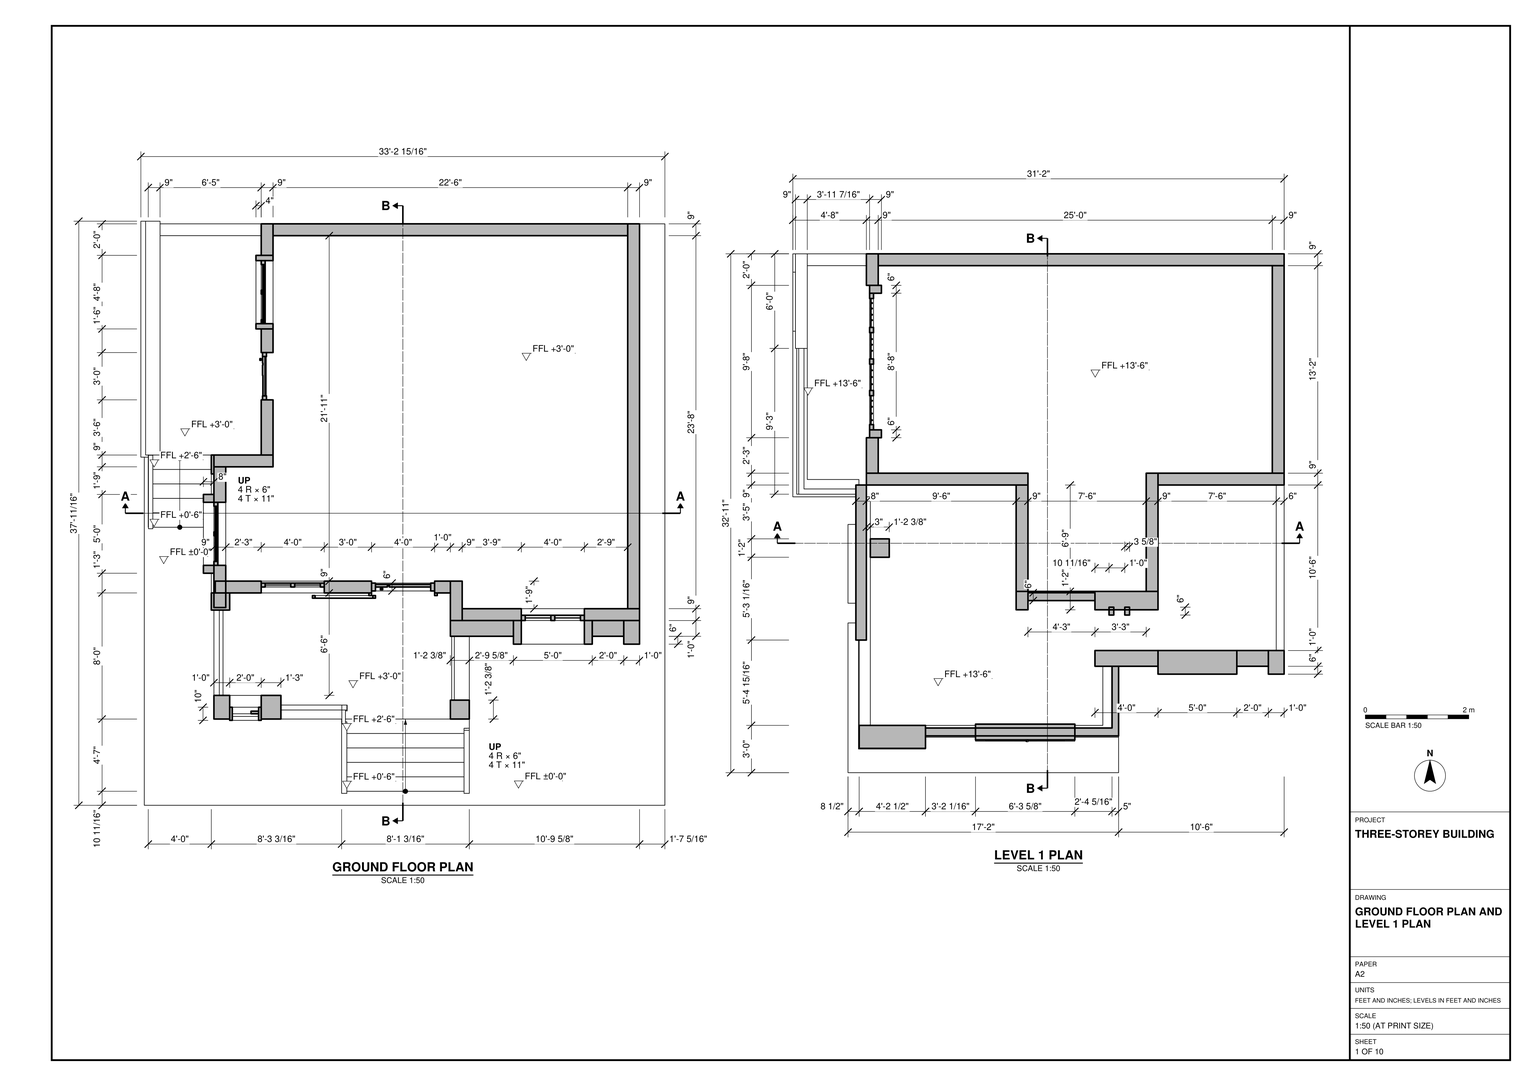
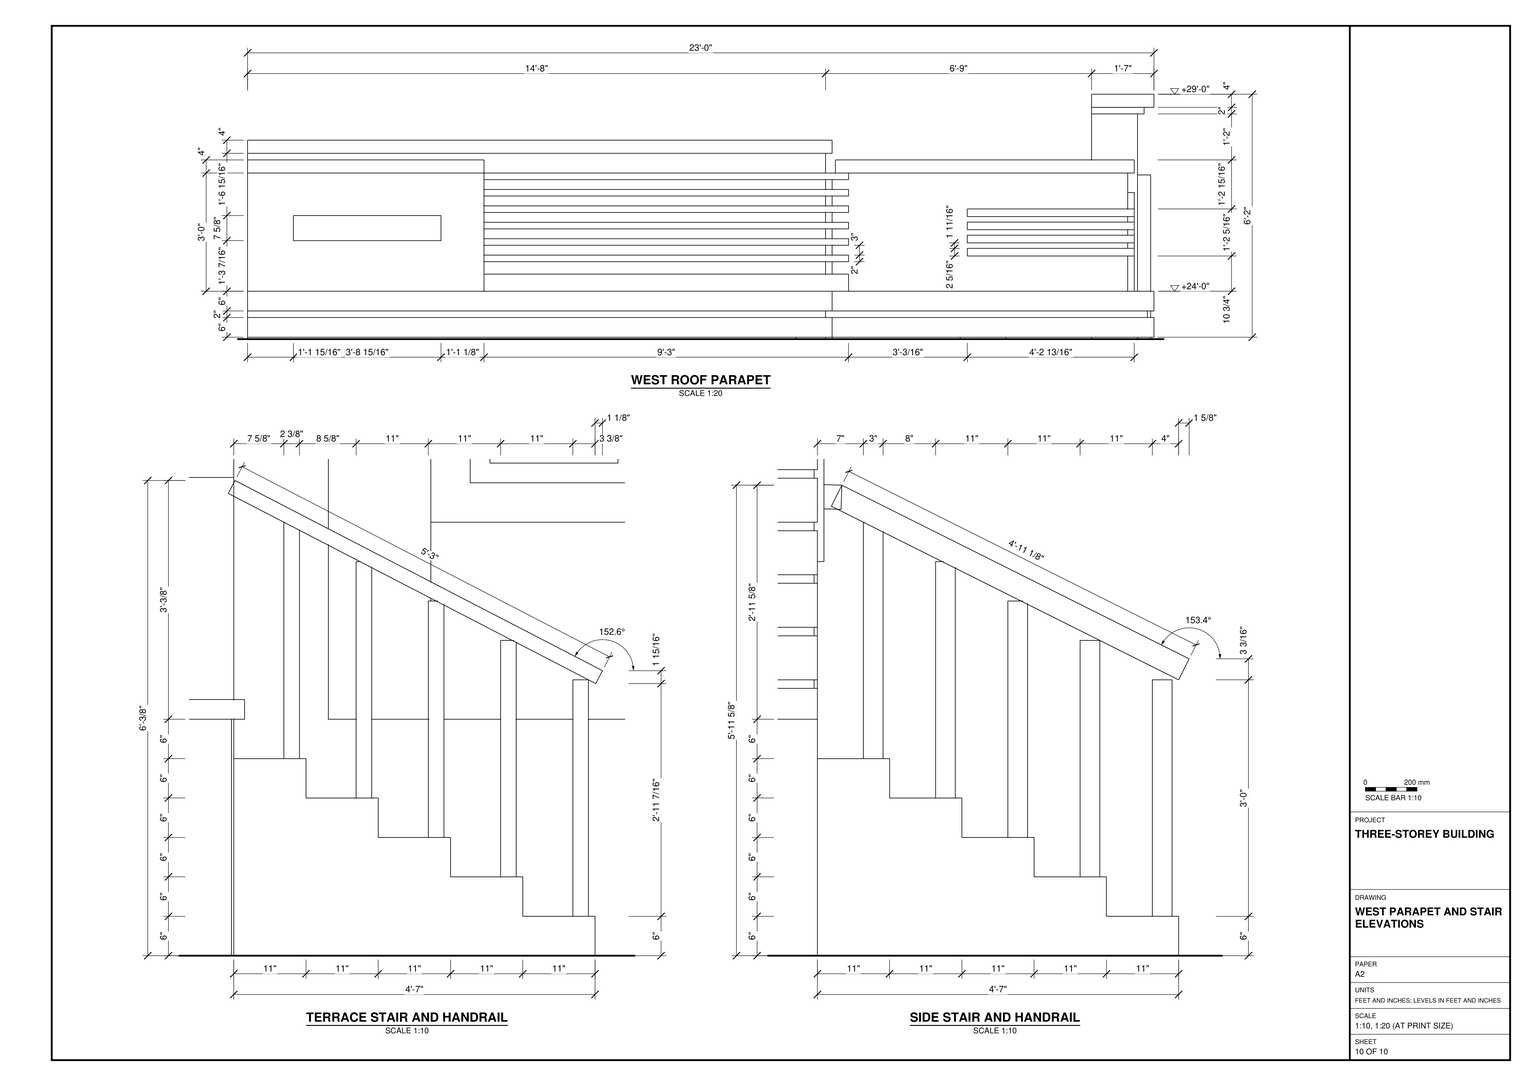
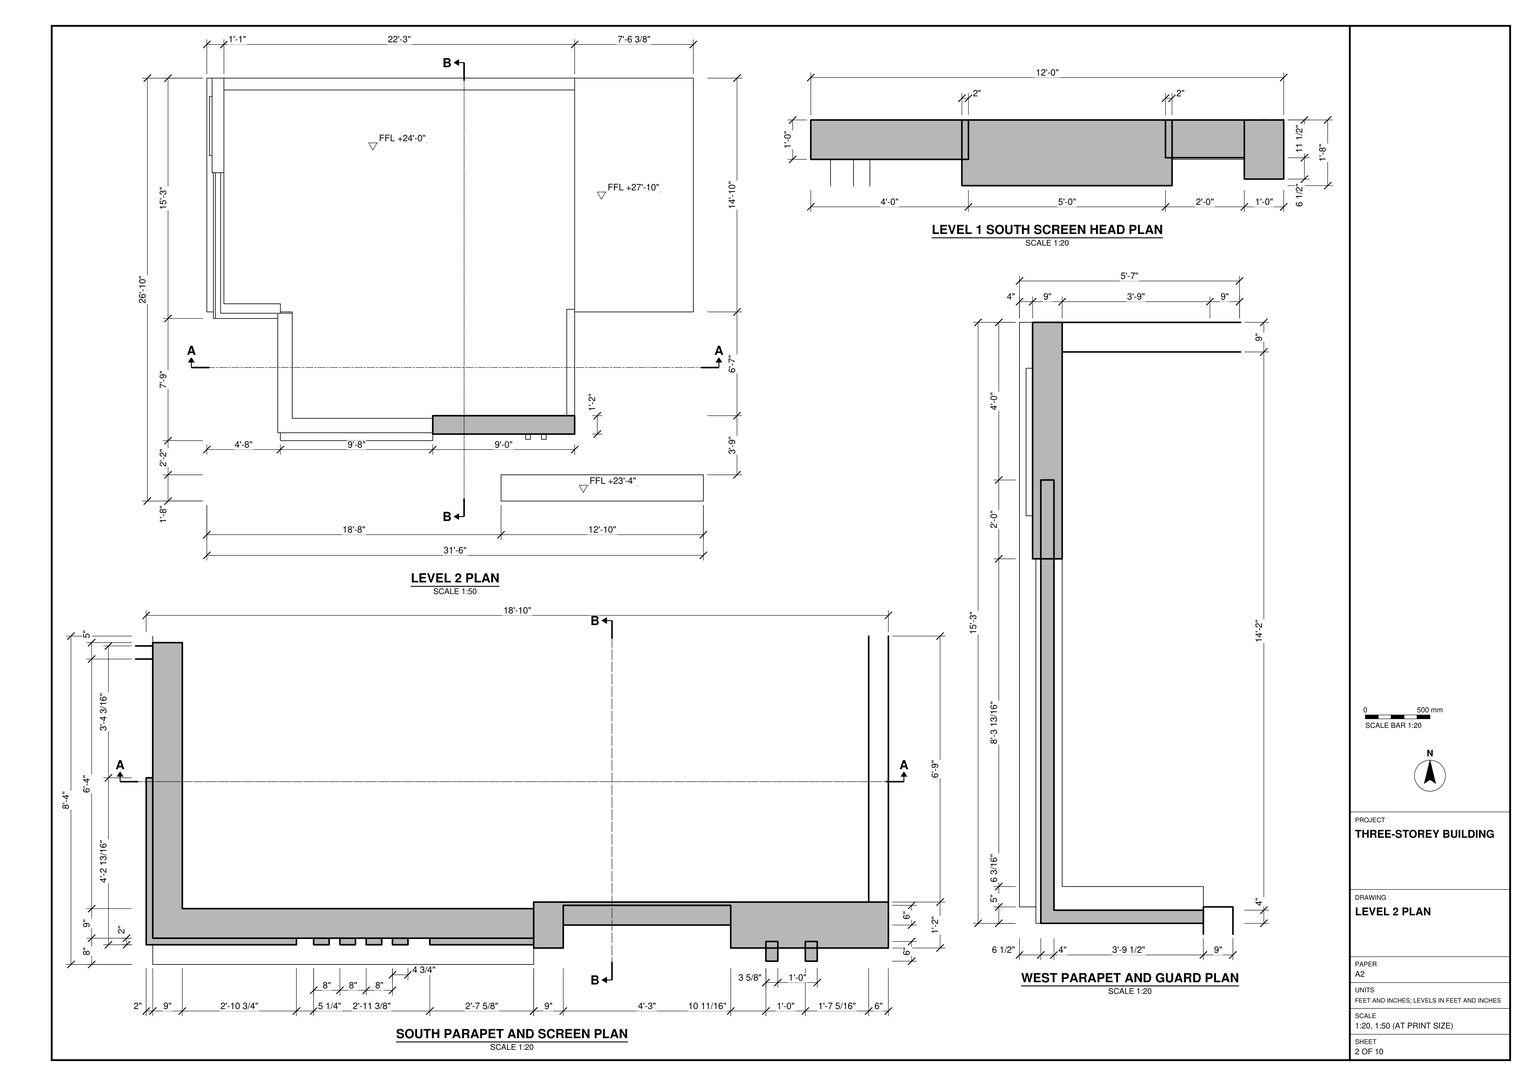
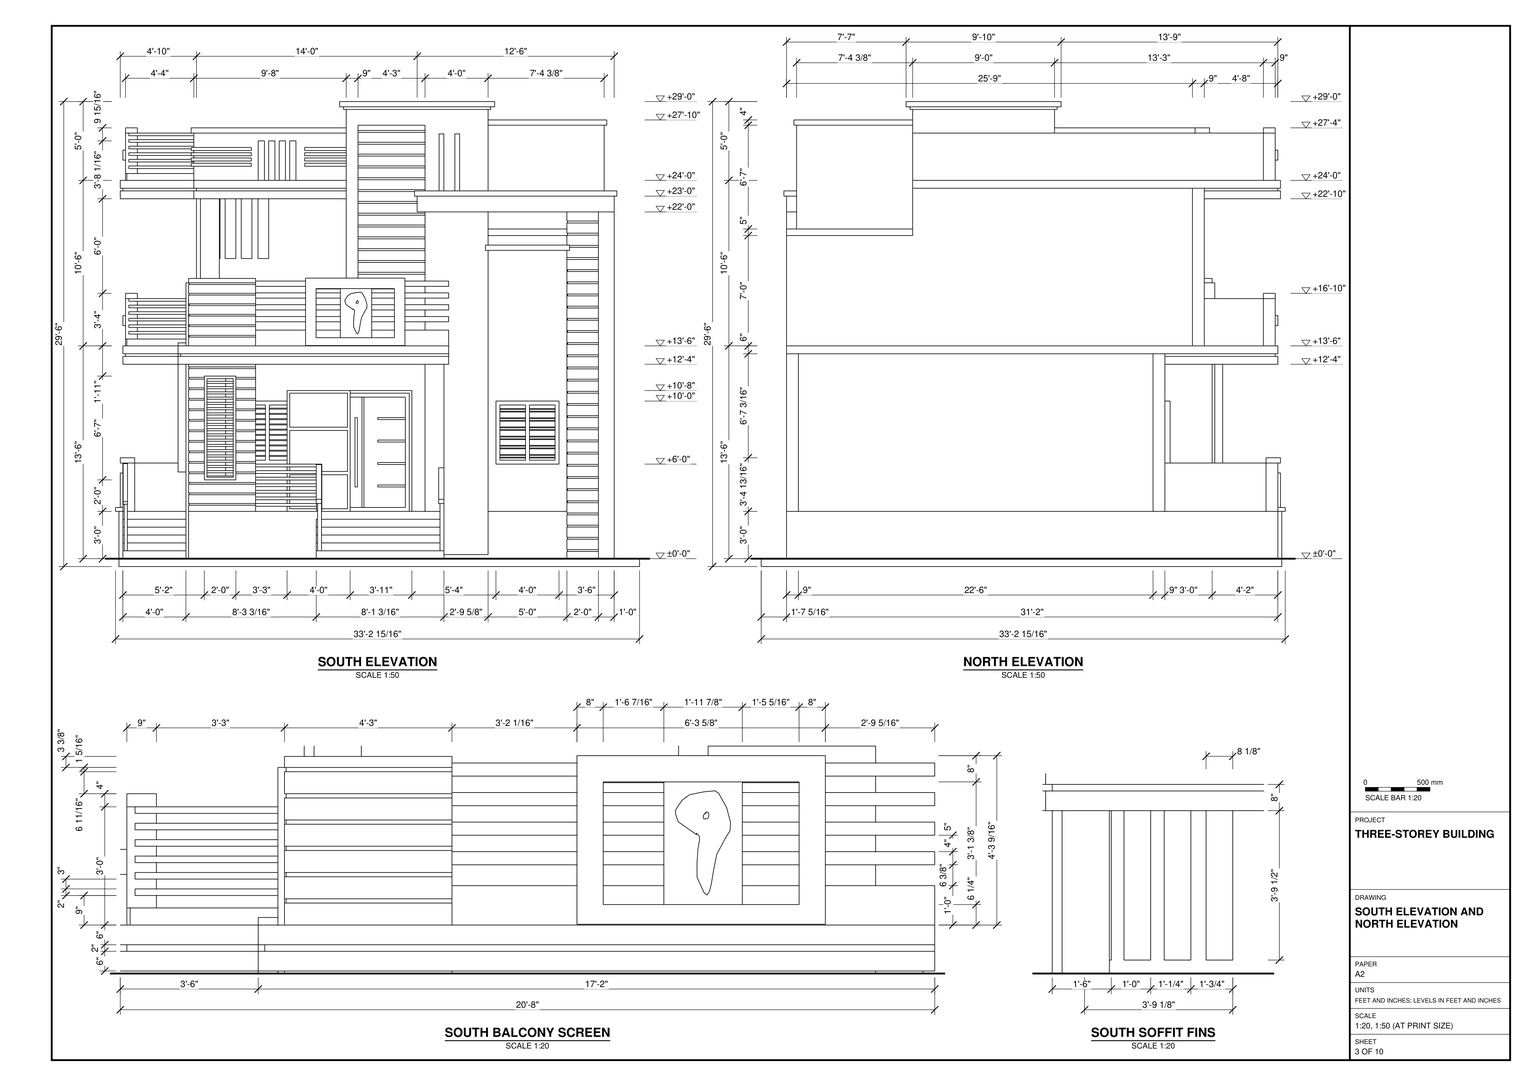
Use task_files/diagram_01.pdf to build the three-storey building in SketchUp. Work in feet and inches. Set the overall dimensions to 33'-2 15/16" along X, 37'-11/16" along Y and 29'-6" along Z. Use ±0'-0" as the ground datum, +13'-6" for level 1 and +24'-0" for level 2. Distinguish the ground datum from the raised ground floor and south terrace at +3'-0".

Follow each plan separately so the wall returns, slab projections and setbacks change at the correct levels. Use the wall thicknesses shown, including the 9" exterior walls, and fit the doors and window units into their openings. Model the south terrace stair and the west side stair with their landings, sloping handrails and upright supports. At level 1, reproduce the projecting south slab, recessed bay and stepped screen head. Follow the level 2 plan for the flat roof surfaces at different heights. Use the parapet details to distinguish solid wall panels from open stretches of horizontal rails.

Keep walls, slabs and roof elements in separate groups or components. Keep each furniture or built-in joinery piece shown separate as well, and use components for repeated parts. Any decor or loose items shown may be suitable library components. Save one SketchUp model as output_files/three_storey_building_with_exterior_stairs_and_parapets.skp.

# SketchUp Ruby script. Lengths in inches.
U = 1.inch
M = Sketchup.active_model
def pt(a) = Geom::Point3d.new(a.map { |v| v * U })
def face(e, loops, mat)
  f = e.add_face(loops[0].map { |a| pt(a) })
  loops[1..].each { |l| e.add_face(l.map { |a| pt(a) }).erase! }
  f.material = f.back_material = mat if mat
  f
end
# faces: each face lists its corners as indices into pts; further lists are holes
def faces(e, pts, list, mat = nil) = list.each { |f| face(e, (f[0].is_a?(Array) ? f : [f]).map { |l| l.map { |i| pts[i] } }, mat) }
# xy, xz, yz: faces in a plane at the given z, y or x. An outline is a flat list of corners, or four numbers for a rectangle; further outlines are holes
def ring(l) = l.size == 4 ? [[l[0], l[1]], [l[2], l[1]], [l[2], l[3]], [l[0], l[3]]] : l.each_slice(2).to_a
def flat(e, list, mat, &to3) = list.each { |f| face(e, (f[0].is_a?(Array) ? f : [f]).map { |l| ring(l).map { |u, v| to3.(u, v) } }, mat) }
def xy(e, z, list, mat = nil) = flat(e, list, mat) { |x, y| [x, y, z] }
def xz(e, y, list, mat = nil) = flat(e, list, mat) { |x, z| [x, y, z] }
def yz(e, x, list, mat = nil) = flat(e, list, mat) { |y, z| [x, y, z] }
def lines(e, pts, list) = list.each { |a, b| e.add_line(pt(pts[a]), pt(pts[b])) }
# prism: a flat outline (further loops are holes) pulled along v
def prism(e, loops, v, mat = nil)
  f = face(e, loops, mat); d = Geom::Vector3d.new(v.map { |x| x * U })
  f.pushpull(f.normal.samedirection?(d) ? d.length : -d.length)
end
def box(e, o, s, mat = nil) = prism(e, [[o, [o[0] + s[0], o[1], o[2]], [o[0] + s[0], o[1] + s[1], o[2]], [o[0], o[1] + s[1], o[2]]]], [0, 0, s[2]], mat)
def at(x, y, z, deg = 0) = Geom::Transformation.translation(pt([x, y, z])) * Geom::Transformation.rotation(ORIGIN, Z_AXIS, deg.degrees)
def axes(o, x, y, z) = Geom::Transformation.new([*x, 0, *y, 0, *z, 0, *pt(o).to_a, 1])
def part(name) = M.definitions.add(name)
# library, detail: a bought-in or finely detailed component or shape, given as its bounding box
def library(name, o, s) = part(name).tap { |d| box(d.entities, o, s) }
def detail(e, o, s) = box(e.add_group.entities, o, s)
def put(e, d, t, mat = nil) = e.add_instance(d, t).tap { |i| i.material = mat if mat }
def group(e, t, mat = nil) = e.add_group.tap { |g| g.transformation = t; g.material = mat if mat }.entities
root = M.entities
M.materials.add("[Color C05]").color = [255, 127, 0]
M.materials.add("[Color C06]").color = [204, 102, 0]
M.materials.add("[Color M00]").color = [255, 255, 255]
M.materials.add("[Color M01]").color = [226, 226, 226]
M.materials.add("[Color M02]").color = [198, 198, 198]
M.materials.add("[Color M05]").color = [114, 114, 114]
M.materials.add("[Color M07]").color = [58, 58, 58]
M.materials.add("[Roofing Slate Tan]").color = [200, 175, 128]
M.materials.add("[Translucent Glass Gray]").color = [128, 128, 128]
M.materials["[Translucent Glass Gray]"].alpha = 0.5
M.materials.add("[Translucent Glass Tinted]").color = [4, 108, 130]
M.materials["[Translucent Glass Tinted]"].alpha = 0.48
M.materials.add("[Wood Cherry Original]").color = [152, 86, 42]
M.materials.add("[Wood Veneer 01]").color = [120, 70, 37]
c1 = part("Group\#14")
box(c1.entities,[0,0,0],[2,93,2])
c2 = part("Group\#29")
prism(c2.entities,[[[0,0.16,0.04],[0,0.09,0.09],[0,0.04,0.16],[0,0.01,0.23],[0,0,0.3125],[0,0.01,0.39],[0,0.04,0.47],[0,0.09,0.53],[0,0.16,0.58],[0,0.23,0.61],[0,0.3125,0.625],[0,0.39,0.61],[0,0.47,0.58],[0,0.53,0.53],[0,0.58,0.47],[0,0.61,0.39],[0,0.625,0.3125],[0,0.61,0.23],[0,0.58,0.16],[0,0.53,0.09],[0,0.47,0.04],[0,0.39,0.01],[0,0.3125,0],[0,0.23,0.01]]],[42,0,0])
c3 = library("Group\#31",[0,0,0],[24,12,228])
c4 = library("Group\#35",[0,0,0],[51,18,177.35])
c5 = part("Group\#37")
box(c5.entities,[0,0,0],[20,2,1.6])
c6 = part("Group\#41")
prism(c6.entities,[[[1.35,42,0.51],[1.28,42,0.34],[1.17,42,0.2],[1.03,42,0.09],[0.87,42,0.02],[0.6875,42,0],[0.51,42,0.02],[0.34,42,0.09],[0.2,42,0.2],[0.09,42,0.34],[0.02,42,0.51],[0,42,0.6875],[0.02,42,0.87],[0.09,42,1.03],[0.2,42,1.17],[0.34,42,1.28],[0.51,42,1.35],[0.6875,42,1.375],[0.87,42,1.35],[1.03,42,1.28],[1.17,42,1.17],[1.28,42,1.03],[1.35,42,0.87],[1.375,42,0.6875]]],[0,-42,0])
c7 = part("Group\#52")
prism(c7.entities,[[[0.5,45,0],[0.37,45,0.02],[0.25,45,0.07],[0.15,45,0.15],[0.07,45,0.25],[0.02,45,0.37],[0,45,0.5],[0.02,45,0.63],[0.07,45,0.75],[0.15,45,0.85],[0.25,45,0.93],[0.37,45,0.98],[0.5,45,1],[0.63,45,0.98],[0.75,45,0.93],[0.85,45,0.85],[0.93,45,0.75],[0.98,45,0.63],[1,45,0.5],[0.98,45,0.37],[0.93,45,0.25],[0.85,45,0.15],[0.75,45,0.07],[0.63,45,0.02]]],[0,-45,0])
c8 = part("Group\#56")
prism(c8.entities,[[[0,0.74,0.28],[0,0.7,0.1875],[0,0.64,0.11],[0,0.5625,0.05],[0,0.47,0.01],[0,0.375,0],[0,0.28,0.01],[0,0.1875,0.05],[0,0.11,0.11],[0,0.05,0.1875],[0,0.01,0.28],[0,0,0.375],[0,0.01,0.47],[0,0.05,0.5625],[0,0.11,0.64],[0,0.1875,0.7],[0,0.28,0.74],[0,0.375,0.75],[0,0.47,0.74],[0,0.5625,0.7],[0,0.64,0.64],[0,0.7,0.5625],[0,0.74,0.47],[0,0.75,0.375]]],[45,0,0])
c9 = part("Group\#66")
prism(c9.entities,[[[0.01,0.31,0],[0.03,0.375,0],[0.07,0.43,0],[0.125,0.47,0],[0.19,0.49,0],[0.25,0.5,0],[0.31,0.49,0],[0.375,0.47,0],[0.43,0.43,0],[0.47,0.375,0],[0.49,0.31,0],[0.5,0.25,0],[0.49,0.19,0],[0.47,0.125,0],[0.43,0.07,0],[0.375,0.03,0],[0.31,0.01,0],[0.25,0,0],[0.19,0.01,0],[0.125,0.03,0],[0.07,0.07,0],[0.03,0.125,0],[0.01,0.19,0],[0,0.25,0]]],[0,0,76])
c10 = part("Group\#109")
prism(c10.entities,[[[0,135,0],[4,135,0],[4,4,0],[43.5,4,0],[43.5,0,0],[0,0,0]]],[0,0,2])
c11 = part("Group\#77")
box(c11.entities,[0,0,0],[9,72,4])
c12 = part("Group\#91")
box(c12.entities,[0,0,0],[8.125,2,45.5])
c13 = part("Group\#93")
prism(c13.entities,[[[0,0,0],[0,6,0],[142,6,0],[142,53,0],[147,53,0],[147,0,0]]],[0,0,4])
c14 = part("Group\#100")
box(c14.entities,[0,0,0],[2,44.9375,7.625])
c15 = part("Group\#111")
prism(c15.entities,[[[2,50.84,0],[2,2,0],[45.75,2,0],[45.75,0,0],[0,0,0],[0,50.84,0]]],[0,0,2.33])
c16 = part("Group\#112")
box(c16.entities,[0,0,0],[31.625,2,2.33])
c17 = part("Group\#113")
box(c17.entities,[0,0,0],[4.73,2,30.0625])
c18 = part("Group\#130")
box(c18.entities,[0,0,0],[50.2,3.75,2.125])
c19 = part("Group\#134")
box(c19.entities,[0,0,0],[2.375,2.375,36])
c20 = part("Group\#139")
box(c20.entities,[0,0,0],[2,6.28,26.23])
box(root,[281.625,120.67,234.73],[64,20,4])
p = [[53.625,259.67,148],[53.625,259.67,154],[253.625,128.67,148],[253.625,128.67,162],[235.625,128.67,162],[235.625,140.67,162],
  [106.625,66.17,162],[106.625,74.67,162]]
lines(root,p,[[0,1],[2,3],[3,4],[4,5],[6,7]])
g1 = group(root,at(55.625,65.67,0))
prism(g1,[[[324,377,0],[324,74.8125,0],[194.4,74.8125,0],[194.4,0,0],[0,0,0],[0,201,0],[-50,201,0],[-50,377,0]]],[0,0,36])
g2 = group(root,at(55.625,161.67,36))
xy(g2,0,[[1,0,120,9],[168,0,180,9]])
xy(g2,36,[[36,0,84,9]])
xy(g2,84,[[36,0,84,9]])
xy(g2,90,[[120,0,168,9]])
xy(g2,120,[[1,0,180,9]])
xz(g2,0,[[[1,0,120,0,120,90,168,90,168,0,180,0,180,120,1,120],[36,36,84,84]]],"[Roofing Slate Tan]")
xz(g2,9,[[[1,0,1,120,180,120,180,0,168,0,168,90,120,90,120,0],[36,36,84,84]]])
yz(g2,1,[[0,0,9,120]])
yz(g2,36,[[0,36,9,84]])
yz(g2,84,[[0,36,9,84]])
yz(g2,120,[[0,0,9,90]])
yz(g2,168,[[0,0,9,90]])
yz(g2,180,[[0,0,9,120]])
g3 = group(root,at(175.625,166.17,36))
prism(g3,[[[48,3,0],[0,3,0],[0,3,90],[48,3,90]],[[45,3,3],[45,3,87],[3,3,87],[3,3,3]]],[0,-6,0],"[Wood Veneer 01]")
g4 = group(root,at(178.625,166.17,39),"[Wood Cherry Original]")
xy(g4,0,[[0,0,0,2,42,2,42,0,10.5,0,10.5,1,9,1,9,0]])
xy(g4,15.6,[[21,0,42,1]])
xy(g4,17.1,[[21,0,42,1]])
xy(g4,32.7,[[21,0,42,1]])
xy(g4,34.2,[[21,0,42,1]])
xy(g4,49.8,[[21,0,42,1]])
xy(g4,51.3,[[21,0,42,1]])
xy(g4,66.9,[[21,0,42,1]])
xy(g4,68.4,[[21,0,42,1]])
xy(g4,84,[[0,0,9,0,9,1,10.5,1,10.5,0,42,0,42,2,0,2]])
xz(g4,0,[[0,0,9,84],[10.5,0,42,0,42,15.6,21,15.6,21,17.1,42,17.1,42,32.7,21,32.7,21,34.2,42,34.2,42,49.8,21,49.8,21,51.3,42,51.3,42,66.9,21,66.9,21,68.4,42,68.4,42,84,10.5,84]])
xz(g4,1,[[9,0,10.5,84],[21,15.6,42,17.1],[21,32.7,42,34.2],[21,49.8,42,51.3],[21,66.9,42,68.4]])
xz(g4,2,[[0,0,42,84]])
yz(g4,0,[[0,0,2,84]])
yz(g4,9,[[0,0,1,84]])
yz(g4,10.5,[[0,0,1,84]])
yz(g4,21,[[0,15.6,1,17.1],[0,32.7,1,34.2],[0,49.8,1,51.3],[0,66.9,1,68.4]])
yz(g4,42,[[0,0,2,0,2,84,0,84,0,68.4,1,68.4,1,66.9,0,66.9,0,51.3,1,51.3,1,49.8,0,49.8,0,34.2,1,34.2,1,32.7,0,32.7,0,17.1,1,17.1,1,15.6,0,15.6]])
g5 = group(root,at(182.3,164.17,54.6))
prism(g5,[[[1.83,2,50.46],[1.83,2,52.8],[1.83,0,52.8],[1.83,0,0],[1.83,2,0],[1.83,2,2.34],[1.83,0.84,2.34],[1.83,0.84,50.46]]],[-1.83,0,0])
g6 = group(root,at(173.625,159.67,36))
prism(g6,[[[2,2,0],[0,2,0],[0,2,92],[52,2,92],[52,2,0],[50,2,0],[50,2,90],[2,2,90]]],[0,-2,0])
g7 = group(root,at(235.625,122.67,36))
box(g7,[0,18,0],[9,30,120],"[Roofing Slate Tan]")
put(root,c1,at(56.125,68.67,30))
g8 = group(root,at(235.625,65.67,36))
box(g8,[0,0,0],[14.4,14.4,120])
g9 = group(root,at(236.625,80.07,70))
box(g9,[0,0,0],[2,48.6,2])
g10 = group(root,at(236.625,80.07,66))
box(g10,[0,0,0],[2,48.6,2])
g11 = group(root,at(236.625,80.07,62))
box(g11,[0,0,0],[2,48.6,2])
g12 = group(root,at(236.625,80.07,58))
box(g12,[0,0,0],[2,48.6,2])
g13 = group(root,at(236.625,80.07,54))
box(g13,[0,0,0],[2,48.6,2])
g14 = group(root,at(236.625,80.07,50))
box(g14,[0,0,0],[2,48.6,2])
g15 = group(root,at(236.625,80.07,46))
box(g15,[0,0,0],[2,48.6,2])
g16 = group(root,at(236.625,80.07,42))
box(g16,[0,0,0],[2,48.6,2])
g17 = group(root,at(236.625,80.07,38))
box(g17,[0,0,0],[2,48.6,2])
g18 = group(root,at(244.625,140.67,36))
prism(g18,[[[0,0,0],[135,0,0],[135,0,120],[0,0,120]],[[93,0,84],[93,0,36],[45,0,36],[45,0,84]]],[0,9,0])
g19 = group(root,at(235.625,128.67,36),"[Color M05]")
box(g19,[0,0,-32.875],[48,12,260.875])
g20 = group(root,at(283.625,122.67,36),"[Color M02]")
prism(g20,[[[0,0,198.73],[0,0,0],[60,0,0],[60,0,198.73]],[[54,0,84],[54,0,36],[6,0,36],[6,0,84]]],[0,18,0])
g21 = group(root,at(289.625,140.67,72),"[Color C06]")
prism(g21,[[[0,4,48],[48,4,48],[48,4,0],[0,4,0]],[[22.5,4,3],[22.5,4,45],[3,4,45],[3,4,3]],[[45,4,45],[25.5,4,45],[25.5,4,3],[45,4,3]]],[0,-4,0])
put(root,c2,at(292.625,142.36,113.64))
put(root,c2,at(292.625,142.36,111.64))
put(root,c2,at(292.625,142.36,104.64))
put(root,c2,at(292.625,142.36,106.64))
put(root,c2,at(292.625,142.36,97.64))
put(root,c2,at(292.625,142.36,99.64))
put(root,c2,at(292.625,142.36,92.64))
put(root,c2,at(292.625,142.36,90.64))
put(root,c2,at(292.625,142.36,85.64))
put(root,c2,at(292.625,142.36,83.64))
put(root,c2,at(292.625,142.36,76.64))
put(root,c2,at(292.625,142.36,78.64))
g22 = group(root,at(292.625,144.67,75),"[Translucent Glass Gray]")
xz(g22,0,[[0,0,42,42]])
put(root,c3,axes([343.625,128.67,0],[1,0,0],[0,1,0],[0,0,1.15789]),"[Color C05]")
g23 = group(root,at(367.625,122.67,36))
xy(g23,-36,[[0,0,12,18]])
xy(g23,228,[[-138,0,0,18],[0,0,12,18]])
xy(g23,240,[[-138,0,12,18]])
xz(g23,0,[[0,-36,12,228],[-138,228,12,240]])
xz(g23,18,[[0,-36,12,228],[-138,228,12,240]])
yz(g23,-138,[[0,228,18,240]])
yz(g23,0,[[0,-36,18,228]])
yz(g23,12,[[0,-36,18,228],[0,228,18,240]])
g24 = group(root,at(59.02,74.67,36))
g25 = group(g24,at(0.7,2.3125,2))
put(g25,c1,axes([0,0,16],[1.41,0,0],[0,0.77031,0],[0,0,1]))
put(g25,c1,axes([0,0,8],[1.41,0,0],[0,0.77031,0],[0,0,1]))
put(g25,c1,axes([0,0,12],[1.41,0,0],[0,0.77031,0],[0,0,1]))
put(g25,c1,axes([0,0,0],[1.41,0,0],[0,0.77031,0],[0,0,1]))
put(g25,c1,axes([0,0,32],[1.41,0,0],[0,0.77031,0],[0,0,1]))
put(g25,c1,axes([0,0,24],[1.41,0,0],[0,0.77031,0],[0,0,1]))
put(g25,c1,axes([0,0,20],[1.41,0,0],[0,0.77031,0],[0,0,1]))
put(g25,c1,axes([0,0,4],[1.41,0,0],[0,0.77031,0],[0,0,1]))
put(g25,c1,axes([0,0,28],[1.41,0,0],[0,0.77031,0],[0,0,1]))
g26 = group(g24,at(0,0,0))
box(g26,[0,0,0],[4.23,2.3125,36])
g27 = group(root,at(55.625,149.67,36),"[Color M02]")
xy(g27,-36,[[-2,-1.05,0,117]])
xy(g27,0,[[0,-1.05,12,12],[-2,12,0,102.6]])
xy(g27,120,[[-2,-1.05,6,12],[6,-1.05,12,12]])
xy(g27,126,[[0,102.6,6,117]])
xy(g27,159.6,[[-2,12,6,102.6]])
xy(g27,174,[[-2,-1.05,6,117]])
xz(g27,-1.05,[[-2,-36,0,-36,0,0,12,0,12,120,-2,120],[-2,120,6,174]])
xz(g27,12,[[-2,0,12,120],[-2,120,6,159.6]])
xz(g27,102.6,[[-2,0,0,0,0,126,6,126,6,159.6,-2,159.6]])
xz(g27,117,[[-2,-36,-2,174,6,174,6,126,0,126,0,-36]])
yz(g27,-2,[[-1.05,-36,-1.05,120,12,120,12,0,102.6,0,102.6,159.6,12,159.6,12,120,-1.05,120,-1.05,174,117,174,117,-36]])
yz(g27,0,[[-1.05,-36,117,-36,117,126,102.6,126,102.6,0,-1.05,0]])
yz(g27,6,[[-1.05,120,12,120,12,159.6,102.6,159.6,102.6,126,117,126,117,174,-1.05,174]])
yz(g27,12,[[-1.05,0,12,120]])
put(root,c4,at(55.625,65.67,36),"[Color C05]")
g28 = group(root,at(67.625,65.67,60))
prism(g28,[[[0,9,0],[0,9,79],[24,9,79],[24,9,0]],[[22,9,2],[22,9,77],[2,9,77],[2,9,2]]],[0,-10,0])
g29 = group(root,at(83.88,72.67,62))
box(g29,[0,-3,0],[5.75,2,75])
put(root,c5,at(69.625,67.67,133.4))
put(root,c5,at(69.625,67.67,129.4))
put(root,c5,at(69.625,67.67,125.4))
put(root,c5,at(69.625,67.67,121.4))
put(root,c5,at(69.625,67.67,117.4))
put(root,c5,at(69.625,67.67,113.4))
put(root,c5,at(69.625,67.67,109.4))
put(root,c5,at(69.625,67.67,105.4))
put(root,c5,at(69.625,67.67,101.4))
put(root,c5,at(69.625,67.67,97.4))
put(root,c5,at(69.625,67.67,93.4))
put(root,c5,at(69.625,67.67,89.4))
put(root,c5,at(69.625,67.67,85.4))
put(root,c5,at(69.625,67.67,81.4))
put(root,c5,at(69.625,67.67,77.4))
put(root,c5,at(69.625,67.67,73.4))
put(root,c5,at(69.625,67.67,69.4))
put(root,c5,at(69.625,67.67,65.4))
put(root,c5,at(69.625,67.67,61.4))
g30 = group(root,at(55.625,182.67,72),"[Color C06]")
prism(g30,[[[3,48,48],[3,0,48],[3,0,0],[3,48,0]],[[3,22.5,45],[3,22.5,3],[3,3,3],[3,3,45]],[[3,25.5,45],[3,45,45],[3,45,3],[3,25.5,3]]],[-3,0,0])
put(root,c6,at(56.4375,185.67,114.06))
put(root,c6,at(56.4375,185.67,110.06))
put(root,c6,at(56.4375,185.67,106.06))
put(root,c6,at(56.4375,185.67,102.06))
put(root,c6,at(56.4375,185.67,98.06))
put(root,c6,at(56.4375,185.67,94.06))
put(root,c6,at(56.4375,185.67,90.06))
put(root,c6,at(56.4375,185.67,86.06))
put(root,c6,at(56.4375,185.67,82.06))
put(root,c6,at(56.4375,185.67,78.06))
g31 = group(root,at(49.625,176.67,36),"[Color M05]")
prism(g31,[[[-2,0,128.31],[-2,60,128.31],[-2,60,30],[-2,0,30]],[[-2,6,36],[-2,54,36],[-2,54,84],[-2,6,84]]],[8,0,0])
g32 = group(root,at(58.625,185.67,75),"[Translucent Glass Gray]")
yz(g32,0,[[0,0,42,42]])
g33 = group(root,at(55.52,176.67,36),"[Color M02]")
box(g33,[0,0,0],[0.1,60,30])
g34 = group(root,at(55.625,257.67,36))
box(g34,[0,0,0],[45,9,120])
g35 = group(root,at(91.625,266.67,36))
prism(g35,[[[9,78,0],[9,176,0],[9,176,120],[9,0,120],[9,0,0],[9,42,0],[9,42,84],[9,78,84]],[[9,152,84],[9,152,36],[9,96,36],[9,96,84]]],[-9,0,0])
g36 = group(root,at(55.625,170.67,36))
xy(g36,0,[[0,-20.11,9,87]])
xy(g36,36,[[0,12,9,60]])
xy(g36,84,[[0,12,9,60]])
xy(g36,112,[[0,-96,9,-20.11]])
xy(g36,126,[[0,-96,0.6,-22.05]])
xy(g36,159.6,[[0.6,-96,9,-96,9,87,0,87,0,-22.05,0.6,-22.05]])
xz(g36,-96,[[0,112,9,112,9,159.6,0.6,159.6,0.6,126,0,126]])
xz(g36,-22.05,[[0,126,0.6,159.6]])
xz(g36,-20.11,[[0,0,9,112]])
xz(g36,12,[[0,36,9,84]])
xz(g36,60,[[0,36,9,84]])
xz(g36,87,[[0,0,9,159.6]])
yz(g36,0,[[[-20.11,0,-20.11,112,-96,112,-96,126,-22.05,126,-22.05,159.6,87,159.6,87,0],[12,36,60,84]]])
yz(g36,0.6,[[-96,126,-22.05,159.6]])
yz(g36,9,[[[-20.11,0,87,0,87,159.6,-96,159.6,-96,112,-20.11,112],[12,36,60,84]]])
p = [[9,-9,126],[6,-9,126]]
lines(g36,p,[[0,1]])
g37 = group(root,at(87.625,362.67,72))
prism(g37,[[[13,56,0],[13,56,48],[13,0,48],[13,0,0]],[[13,52,4],[13,4,4],[13,4,44],[13,52,44]]],[-13,0,0])
g38 = group(root,at(91.625,366.67,76),"[Color C06]")
prism(g38,[[[3,48,40],[3,0,40],[3,0,0],[3,48,0]],[[3,22.5,37],[3,22.5,3],[3,3,3],[3,3,37]],[[3,25.5,37],[3,45,37],[3,45,3],[3,25.5,3]]],[-3,0,0])
put(root,c7,at(92.625,366.67,110.41))
put(root,c7,at(92.625,366.67,106.41))
put(root,c7,at(92.625,366.67,102.41))
put(root,c7,at(92.625,366.67,98.41))
put(root,c7,at(92.625,366.67,94.41))
put(root,c7,at(92.625,366.67,90.41))
put(root,c7,at(92.625,366.67,86.41))
put(root,c7,at(92.625,366.67,82.41))
put(root,c7,at(92.625,366.67,74.41))
g39 = group(root,at(94.625,369.67,79),"[Translucent Glass Gray]")
yz(g39,0,[[0,0,42,34]])
g40 = group(root,at(130.625,157.67,36),"[Wood Cherry Original]")
g41 = group(g40,at(2,0,2),"[Translucent Glass Tinted]")
xz(g41,0,[[0,0,44,25.9]])
g42 = group(g40,at(0,0,0))
prism(g42,[[[48,2,0],[0,2,0],[0,2,92],[48,2,92]],[[46,2,30.4],[46,2,61.6],[2,2,61.6],[2,2,30.4]],[[2,2,90],[2,2,64.1],[46,2,64.1],[46,2,90]],[[46,2,2],[46,2,27.9],[2,2,27.9],[2,2,2]]],[0,-2,0])
g43 = group(g40,at(2,0,30.4),"[Translucent Glass Tinted]")
xz(g43,0,[[0,0,44,31.2]])
g44 = group(g40,at(2,0,64.1),"[Translucent Glass Tinted]")
xz(g44,0,[[0,0,44,25.9]])
g45 = group(root,at(91.625,166.17,72),"[Color C06]")
prism(g45,[[[0,3,48],[48,3,48],[48,3,0],[0,3,0]],[[22.5,3,3],[22.5,3,45],[3,3,45],[3,3,3]],[[45,3,45],[25.5,3,45],[25.5,3,3],[45,3,3]]],[0,-3,0])
put(root,c8,at(94.625,167.3,113.84))
put(root,c8,at(94.625,167.3,109.84))
put(root,c8,at(94.625,167.3,105.84))
put(root,c8,at(94.625,167.3,101.84))
put(root,c8,at(94.625,167.3,97.84))
put(root,c8,at(94.625,167.3,93.84))
put(root,c8,at(94.625,167.3,89.84))
put(root,c8,at(94.625,167.3,85.84))
put(root,c8,at(94.625,167.3,81.84))
put(root,c8,at(94.625,167.3,77.84))
g46 = group(root,at(94.625,169.17,75),"[Translucent Glass Gray]")
xz(g46,0,[[0,0,42,42]])
g47 = group(root,at(90.625,308.67,36),"[Wood Veneer 01]")
g48 = group(g47,at(2,0,0))
prism(g48,[[[3,0,0],[3,36,0],[3,36,84],[3,0,84]],[[3,3,81],[3,33,81],[3,33,3],[3,3,3]]],[-3,0,0])
g49 = group(g47,at(2,3,3))
xy(g49,0,[[0,0,0,23.5,0.3,23.5,0.3,25,0,25,0,30,2,30,2,0]])
xy(g49,6.9,[[0,0,0.3,15.6]])
xy(g49,8.4,[[0,0,0.3,15.6]])
xy(g49,24.9,[[0,0,0.3,15.6]])
xy(g49,26.4,[[0,0,0.3,15.6]])
xy(g49,42.9,[[0,0,0.3,15.6]])
xy(g49,44.4,[[0,0,0.3,15.6]])
xy(g49,60.9,[[0,0,0.3,15.6]])
xy(g49,62.4,[[0,0,0.3,15.6]])
xy(g49,78,[[0,0,2,0,2,30,0,30,0,25,0.3,25,0.3,23.5,0,23.5]])
xz(g49,0,[[0,0,2,0,2,78,0,78,0,62.4,0.3,62.4,0.3,60.9,0,60.9,0,44.4,0.3,44.4,0.3,42.9,0,42.9,0,26.4,0.3,26.4,0.3,24.9,0,24.9,0,8.4,0.3,8.4,0.3,6.9,0,6.9]])
xz(g49,15.6,[[0,6.9,0.3,8.4],[0,24.9,0.3,26.4],[0,42.9,0.3,44.4],[0,60.9,0.3,62.4]])
xz(g49,23.5,[[0,0,0.3,78]])
xz(g49,25,[[0,0,0.3,78]])
xz(g49,30,[[0,0,2,78]])
yz(g49,0,[[0,0,0,6.9,15.6,6.9,15.6,8.4,0,8.4,0,24.9,15.6,24.9,15.6,26.4,0,26.4,0,42.9,15.6,42.9,15.6,44.4,0,44.4,0,60.9,15.6,60.9,15.6,62.4,0,62.4,0,78,23.5,78,23.5,0],[25,0,30,78]])
yz(g49,0.3,[[23.5,0,25,78],[0,6.9,15.6,8.4],[0,24.9,15.6,26.4],[0,42.9,15.6,44.4],[0,60.9,15.6,62.4]])
yz(g49,2,[[0,0,30,78]])
g50 = group(g47,at(0,30.09,21.01))
prism(g50,[[[2,0,0],[2,0,1.78],[0.78,0,1.78],[0.78,0,38.29],[2,0,38.29],[2,0,40.0625],[0,0,40.0625],[0,0,0]]],[0,1.3125,0])
g51 = group(root,at(370.625,149.67,36))
box(g51,[0,0,0],[9,293,120])
g52 = group(root,at(100.625,433.67,36))
box(g52,[0,0,0],[270,9,120])
g53 = group(root,at(100.625,149.67,156))
prism(g53,[[[279,293,0],[279,-9,0],[153,-9,0],[153,-102,0],[-53,-102,0],[-53,12,0],[-39,12,0],[-39,117,0],[-47,117,0],[-47,108,0],[-95,108,0],[-95,293,0]]],[0,0,6])
g54 = group(root,at(67.625,65.67,148))
xy(g54,0,[[-20,-18,186,96]])
xy(g54,6,[[-20,-18,186,-16],[-20,-16,-18,96],[-18,-16,186,96]])
xy(g54,8,[[-18,-16,186,96]])
xz(g54,-18,[[-20,0,186,6]])
xz(g54,-16,[[-18,6,186,8]])
xz(g54,96,[[-20,0,186,6],[-18,6,186,8]])
yz(g54,-20,[[-18,0,96,6]])
yz(g54,-18,[[-16,6,96,8]])
yz(g54,186,[[-18,0,96,6],[-16,6,96,8]])
g55 = group(root,at(61.625,266.67,162),"[Color M00]")
prism(g55,[[[9,9,0],[9,36,0],[9,36,90],[9,152,90],[9,152,0],[9,176,0],[9,176,120],[9,9,120]]],[-9,0,0])
g56 = group(root,at(64.0625,302.67,162))
prism(g56,[[[9,6,0],[9,6,84],[9,110,84],[9,110,0],[9,116,0],[9,116,90],[9,0,90],[9,0,0]]],[-9,0,0])
g57 = group(root,at(64.0625,308.67,162),"[Color C06]")
prism(g57,[[[3,104,84],[3,0,84],[3,0,0],[3,104,0]],[[3,26,80],[3,26,4],[3,4,4],[3,4,80]],[[3,78,80],[3,100,80],[3,100,4],[3,78,4]],[[3,74,80],[3,74,4],[3,54,4],[3,54,80]],[[3,50,4],[3,30,4],[3,30,80],[3,50,80]]],[-3,0,0])
put(root,c9,at(65.6,404.9375,166))
put(root,c9,at(65.6,400.8125,166))
put(root,c9,at(65.6,396.0625,166))
put(root,c9,at(65.6,391.9375,166))
put(root,c9,at(65.6,377.5,166))
put(root,c9,at(65.6,373.25,166))
put(root,c9,at(65.6,368.625,166))
put(root,c9,at(65.6,353.75,166))
put(root,c9,at(65.6,348.6,166))
put(root,c9,at(65.6,343.16,166))
put(root,c9,at(65.6,330.6,166),"[Translucent Glass Gray]")
put(root,c9,at(65.6,325.97,166))
put(root,c9,at(65.6,320.85,166))
put(root,c9,at(65.6,315.78,166))
g58 = group(root,at(65.0625,312.67,166),"[Translucent Glass Gray]")
yz(g58,0,[[0,0,22,76]])
g59 = group(root,at(65.0625,338.67,166),"[Translucent Glass Gray]")
yz(g59,0,[[0,0,20,76]])
g60 = group(root,at(65.0625,362.67,166),"[Translucent Glass Gray]")
yz(g60,0,[[0,0,20,76]])
g61 = group(root,at(65.0625,386.67,166),"[Translucent Glass Gray]")
yz(g61,0,[[0,0,22,76]])
g62 = group(root,at(61.625,266.67,162))
box(g62,[0,0,0],[123,9,120])
g63 = group(root,at(7.625,266.67,148))
xy(g63,0,[[-2,-9,84,176]])
xy(g63,6,[[-2,-9,46,-9,46,-7,0,-7,0,-5,-2,-5],[46,-9,84,0],[0,-7,46,-7,46,0,84,0,84,176,0,176],[-2,-5,0,176]])
xy(g63,8,[[0,-7,46,-7,46,0,84,0,84,176,0,176]])
xz(g63,-9,[[-2,0,84,6]])
xz(g63,-7,[[0,6,46,8]])
xz(g63,0,[[46,6,84,8]])
xz(g63,176,[[-2,0,84,6],[0,6,84,8]])
yz(g63,-2,[[-9,0,176,6]])
yz(g63,0,[[-7,6,176,8]])
yz(g63,46,[[-7,6,0,8]])
yz(g63,84,[[-9,0,176,6],[0,6,176,8]])
p = [[46,0,6],[46,0,0.0625]]
lines(g63,p,[[0,1]])
put(root,c10,at(10.125,259.67,196))
put(root,c10,at(10.125,259.67,191))
put(root,c10,at(10.125,259.67,186))
put(root,c10,at(10.125,259.67,181))
put(root,c10,at(10.125,259.67,176))
put(root,c10,at(10.125,259.67,171))
g64 = group(root,at(10.125,259.67,156))
xy(g64,0,[[0,0,0,135,4,135,4,4,43.5,4,43.5,0]])
xz(g64,4,[[4,0,43.5,2]])
xz(g64,135,[[0,0,4,2]])
yz(g64,0,[[0,0,135,2]])
yz(g64,4,[[4,0,135,2]])
yz(g64,43.5,[[0,0,4,2]])
g65 = group(root,at(64.625,211.67,162))
box(g65,[0,0,0],[14.4,14,120])
g66 = group(root,at(175.625,185.67,162))
box(g66,[0,0,0],[9,81,120])
g67 = group(root,at(175.625,176.67,162),"[Color M01]")
xy(g67,0,[[0,-5,0,9,108,9,108,-5,60,-5,60,8,9,8,9,-5]])
xy(g67,168,[[9,-5,60,8]])
xy(g67,180,[[0,-5,108,9]])
xz(g67,-5,[[0,0,9,0,9,168,60,168,60,0,108,0,108,180,0,180]])
xz(g67,8,[[9,0,60,168]])
xz(g67,9,[[0,0,108,180]])
yz(g67,0,[[-5,0,9,180]])
yz(g67,9,[[-5,0,8,168]])
yz(g67,60,[[-5,0,8,168]])
yz(g67,108,[[-5,0,9,180]])
put(root,c11,at(7.625,370.67,198))
g68 = group(root,at(7.625,394.67,162),"[Color M05]")
xy(g68,0,[[1,-135,1,-24,0,-24,0,48,9,48,9,-123.8,48.3125,-123.8,48.3125,-135]])
xy(g68,5.21,[[1,-135,48.3125,-135,48.3125,-123.8,9,-123.8,9,-24,1,-24]],"[Color M01]")
xy(g68,36,[[0,-24,9,48]])
xz(g68,-135,[[1,0,48.3125,5.21]],"[Color M01]")
xz(g68,-123.8,[[9,0,48.3125,5.21]])
xz(g68,-24,[[0,0,1,5.21],[0,5.21,9,36]])
xz(g68,48,[[0,0,9,36]])
yz(g68,0,[[-24,0,48,36]])
yz(g68,1,[[-135,0,-24,5.21]],"[Color M01]")
yz(g68,9,[[-123.8,0,48,0,48,36,-24,36,-24,5.21,-123.8,5.21]])
yz(g68,48.3125,[[-135,0,-123.8,5.21]])
g69 = group(root,at(16.625,433.67,162))
box(g69,[0,0,0],[45,9,36])
g70 = group(root,at(184.625,178.67,162),"[Color C05]")
prism(g70,[[[0,6,168],[0,6,0],[0,0,0],[0,0,9.5],[0,0.5,9.5],[0,0.5,11],[0,0,11],[0,0,18.5],[0,0.5,18.5],[0,0.5,20],[0,0,20],[0,0,27.5],[0,0.5,27.5],[0,0.5,29],[0,0,29],[0,0,36.5],[0,0.5,36.5],[0,0.5,38],[0,0,38],[0,0,45.5],[0,0.5,45.5],[0,0.5,47],[0,0,47],[0,0,54.5],[0,0.5,54.5],[0,0.5,56],[0,0,56],[0,0,63.5],[0,0.5,63.5],[0,0.5,65],[0,0,65],[0,0,72.5],[0,0.5,72.5],[0,0.5,74],[0,0,74],[0,0,81.5],[0,0.5,81.5],[0,0.5,83],[0,0,83],[0,0,90.5],[0,0.5,90.5],[0,0.5,92],[0,0,92],[0,0,99.5],[0,0.5,99.5],[0,0.5,101],[0,0,101],[0,0,108.5],[0,0.5,108.5],[0,0.5,110],[0,0,110],[0,0,117.5],[0,0.5,117.5],[0,0.5,119],[0,0,119],[0,0,126.5],[0,0.5,126.5],[0,0.5,128],[0,0,128],[0,0,135.5],[0,0.5,135.5],[0,0.5,137],[0,0,137],[0,0,144.5],[0,0.5,144.5],[0,0.5,146],[0,0,146],[0,0,153.5],[0,0.5,153.5],[0,0.5,155],[0,0,155],[0,0,162.5],[0,0.5,162.5],[0,0.5,164],[0,0,164],[0,0,168]]],[51,0,0])
g71 = group(root,at(274.625,185.67,162))
box(g71,[0,0,0],[9,90,120])
g72 = group(root,at(283.625,266.67,162))
box(g72,[0,0,0],[96,9,84])
g73 = group(root,at(70.625,433.67,162))
prism(g73,[[[0,0,0],[309,0,0],[309,0,84],[213,0,84],[213,0,120],[0,0,120]]],[0,9,0])
g74 = group(root,at(370.625,266.67,162))
box(g74,[0,9,0],[9,158,84])
g75 = group(root,at(61.625,176.67,274))
xy(g75,0,[[-2,-10,114,90]])
xy(g75,6,[[-2,-10,114,-10,114,-8,0,-8,0,0,-2,0],[0,-8,114,90],[-2,0,0,90]])
xy(g75,8,[[0,-8,114,90]])
xz(g75,-10,[[-2,0,114,6]],"[Color M05]")
xz(g75,-8,[[0,6,114,8]],"[Color M07]")
xz(g75,90,[[-2,0,114,6],[0,6,114,8]])
yz(g75,-2,[[-10,0,90,6]],"[Color M05]")
yz(g75,0,[[-8,6,90,8]],"[Color M07]")
yz(g75,114,[[-10,0,90,6],[-8,6,90,8]])
g76 = group(root,at(61.625,176.67,282))
xy(g76,0,[[-2,-10,-2,88,-58,88,-58,266,222,266,222,9,114,9,114,-10]])
xy(g76,6,[[-2,-10,114,-10,114,9,222,9,222,266,-58,266,-58,88,-2,88]])
xz(g76,-10,[[-2,0,114,6]],"[Color M05]")
xz(g76,9,[[114,0,222,6]])
xz(g76,88,[[-58,0,-2,6]])
xz(g76,266,[[-58,0,222,6]])
yz(g76,-58,[[88,0,266,6]])
yz(g76,-2,[[-10,0,88,6]],"[Color M05]")
yz(g76,114,[[-10,0,9,6]])
yz(g76,222,[[9,0,90,6],[90,0,266,6]])
g77 = group(root,at(5.625,266.67,274))
xy(g77,0,[[-2,-2,56,176]])
xy(g77,6,[[-2,-2,0,176],[0,-2,56,0],[0,0,56,176]])
xy(g77,8,[[0,0,56,176]])
xz(g77,-2,[[-2,0,56,6]])
xz(g77,0,[[0,6,56,8]])
xz(g77,176,[[-2,0,56,6],[0,6,56,8]])
yz(g77,-2,[[-2,0,176,6]])
yz(g77,0,[[0,6,176,8]])
yz(g77,56,[[-2,0,176,6],[0,6,176,8]])
g78 = group(root,at(283.625,266.67,246))
box(g78,[0,0,0],[96,176,5])
g79 = group(root,at(283.625,266.67,251),"[Color M02]")
box(g79,[0,0,0],[88.36,176,79])
put(root,c12,at(71.47,264.67,228.5),"[Roofing Slate Tan]")
put(root,c12,at(83.47,264.67,228.5),"[Roofing Slate Tan]")
g80 = group(root,at(106.625,74.67,162))
prism(g80,[[[147,0,0],[0,0,0],[0,9,0],[135,9,0],[135,54,0],[147,54,0]]],[0,0,12])
put(root,c13,at(106.625,75.67,207.35))
put(root,c13,at(106.625,75.67,198.35))
put(root,c13,at(106.625,75.67,189.35))
put(root,c13,at(106.625,75.67,180.35))
g81 = group(root,at(150.68,71.67,162))
prism(g81,[[[-6,12,0],[-6,13.04,51.35],[69.64,13.04,51.35],[69.64,12,0]],[[2,12.12,6],[61.64,12.12,6],[61.64,12.875,43.35],[2,12.875,43.35]]],[0,-12,0.24])
g82 = group(root,at(171.14,73.17,168.24),"[Color M01]")
box(g82,[0,0,0],[23.9,10,37.35])
g83 = group(root,at(227.625,120.67,276),"[Color M05]")
box(g83,[0,0,0],[154,20,4])
g84 = group(root,at(175.625,176.67,342))
box(g84,[-2,-7,0],[112,16,2])
g85 = group(root,at(172.625,173.67,344))
box(g85,[-2,-7,0],[118,19,4])
g86 = group(root,at(246.34,171.67,169.42))
box(g86,[0,-4,0],[3.625,6,154])
g87 = group(root,at(258.34,171.67,169.42))
box(g87,[0,-4,0],[3.625,6,154])
put(root,c14,at(5.625,383.77,177.42))
g88 = group(root,at(10.125,259.67,297))
prism(g88,[[[0,135,0],[4,135,0],[4,4,0],[49.5,4,0],[49.5,0,0],[0,0,0]]],[0,0,2])
put(root,c11,at(7.625,370.67,324))
g89 = group(root,at(7.625,394.67,288),"[Color M02]")
xy(g89,0,[[1,-135,1,-24,0,-24,0,48,9,48,9,-123.8,52,-123.8,52,-135]])
xy(g89,5.21,[[1,-135,52,-135,52,-123.8,9,-123.8,9,-24,1,-24]])
xy(g89,36,[[0,-24,9,48]])
xz(g89,-135,[[1,0,52,5.21]])
xz(g89,-123.8,[[9,0,52,5.21]])
xz(g89,-24,[[0,0,1,5.21],[0,5.21,9,36]])
xz(g89,48,[[0,0,9,36]],"[Color M05]")
yz(g89,0,[[-24,0,48,36]],"[Color M05]")
yz(g89,1,[[-135,0,-24,5.21]])
yz(g89,9,[[-123.8,0,48,0,48,36,-24,36,-24,5.21,-123.8,5.21]])
yz(g89,52,[[-135,0,-123.8,5.21]])
g90 = group(root,at(16.625,433.67,288))
box(g90,[0,0,0],[267,9,36])
put(root,c14,at(5.625,383.77,303.42))
g91 = group(root,at(10.125,259.67,307))
prism(g91,[[[0,135,0],[4,135,0],[4,4,0],[49.5,4,0],[49.5,0,0],[0,0,0]]],[0,0,2])
g92 = group(root,at(10.125,259.67,302))
prism(g92,[[[0,135,0],[4,135,0],[4,4,0],[49.5,4,0],[49.5,0,0],[0,0,0]]],[0,0,2])
g93 = group(root,at(10.125,259.67,312))
prism(g93,[[[0,135,0],[4,135,0],[4,4,0],[49.5,4,0],[49.5,0,0],[0,0,0]]],[0,0,2])
g94 = group(root,at(10.125,259.67,317))
prism(g94,[[[0,135,0],[4,135,0],[4,4,0],[49.5,4,0],[49.5,0,0],[0,0,0]]],[0,0,2])
g95 = group(root,at(10.125,259.67,322))
prism(g95,[[[0,135,0],[4,135,0],[4,4,0],[49.5,4,0],[49.5,0,0],[0,0,0]]],[0,0,2])
g96 = group(root,at(59.625,174.67,288))
prism(g96,[[[116,0,0],[0,0,0],[0,90,0],[9,90,0],[9,9,0],[116,9,0]]],[0,0,36])
put(root,c15,at(57.625,172.67,310.74),"[Color M05]")
put(root,c15,at(57.625,172.67,306.74),"[Color M05]")
put(root,c15,at(57.625,172.67,302.74),"[Color M05]")
put(root,c15,at(57.625,172.67,298.74),"[Color M05]")
put(root,c16,at(144,172.67,310.74),"[Color M05]")
put(root,c16,at(144,172.67,306.74),"[Color M05]")
put(root,c16,at(144,172.67,302.74),"[Color M05]")
put(root,c16,at(144,172.67,298.74),"[Color M05]")
put(root,c17,at(108.62,172.67,288))
put(root,c17,at(116.62,172.67,288))
put(root,c17,at(124.62,172.67,288))
put(root,c17,at(132.62,172.67,288))
g97 = group(root,at(57.625,172.67,324))
prism(g97,[[[0,91,0],[11,91,0],[11,11,0],[118,11,0],[118,0,0],[0,0,0]]],[0,0,4])
put(root,c12,at(95.72,264.67,228.5),"[Roofing Slate Tan]")
put(root,c12,at(108.47,264.67,228.5),"[Roofing Slate Tan]")
g98 = group(root,at(373.625,140.67,162))
box(g98,[0,0,0],[6,126,36])
g99 = group(root,at(-3.45,-88.9375,-6))
box(g99,[6.07,88.9375,0],[396.3,442.67,6])
g100 = group(root,at(152.83,10.67,0),"[Color M07]")
prism(g100,[[[97.2,55,0],[97.2,55,30],[97.2,44,30],[97.2,44,24],[97.2,33,24],[97.2,33,18],[97.2,22,18],[97.2,22,12],[97.2,11,12],[97.2,11,6],[97.2,0,6],[97.2,0,0]]],[-97.2,0,0])
p = [[97.2,55,36],[97.2,55,30]]
lines(g100,p,[[0,1]])
g101 = group(root,at(152.83,10.67,6))
box(g101,[1,1,0],[3,3,36])
g102 = group(root,at(246.02,10.67,6))
box(g102,[1,1,0],[3,3,36])
g103 = group(root,at(246.02,21.67,12))
box(g103,[1,1,0],[3,3,36])
g104 = group(root,at(246.02,32.67,18))
box(g104,[1,1,0],[3,3,36])
g105 = group(root,at(246.02,43.67,24))
box(g105,[1,1,0],[3,3,36])
g106 = group(root,at(246.02,54.67,30))
box(g106,[1,1,0],[3,3,36])
g107 = group(root,at(152.83,9.07,42))
prism(g107,[[[0,1.6,0],[0,0,3.2],[4,0,3.2],[4,1.6,0],[2,1.6,0]]],[0,52.87,26.4375])
g108 = group(root,at(246.02,9.07,42))
prism(g108,[[[0,1.6,0],[0,0,3.2],[4,0,3.2],[4,1.6,0],[2,1.6,0]]],[0,48,24])
g109 = group(root,at(152.83,21.67,12))
box(g109,[1,1,0],[3,3,36])
g110 = group(root,at(152.83,54.67,30))
box(g110,[1,1,0],[3,3,36])
g111 = group(root,at(152.83,43.67,24))
box(g111,[1,1,0],[3,3,36])
g112 = group(root,at(152.83,32.67,18))
box(g112,[1,1,0],[3,3,36])
put(root,c18,at(106.625,72.5625,69.875))
put(root,c18,at(106.625,72.5625,64.875))
put(root,c18,at(106.625,72.5625,59.875))
put(root,c18,at(106.625,72.5625,54.875))
put(root,c18,at(106.625,72.5625,49.875))
put(root,c18,at(106.625,72.5625,44.875))
put(root,c18,at(106.625,72.5625,39.875))
g113 = group(root,at(153.01,61.94,36.875))
xy(g113,0,[[0,9.93,4.0625,14.37]])
xy(g113,31.43,[[0,9.93,2.75,10.62]])
xy(g113,35.125,[[2.75,9.93,4.0625,9.93,4.0625,14.37,0,14.37,0,10.62,2.75,10.62]])
xz(g113,9.93,[[0,0,4.0625,0,4.0625,35.125,2.75,35.125,2.75,31.43,0,31.43]])
xz(g113,10.62,[[2.75,31.43,3.8125,35.125]])
xz(g113,14.37,[[0,0,4.0625,35.125]])
yz(g113,0,[[9.93,0,9.93,31.41,10.62,31.43,10.75,31.4375,10.62,35.125,14.37,35.125,14.37,0],[0.125,31.07,0,34.76,10.62,35.125,10.75,31.4375,10.62,31.43,9.93,31.43,9.93,31.41],[9.93,31.41,9.93,31.43,10.62,31.43]])
yz(g113,2.75,[[0.125,31.07,10.62,31.43,9.93,31.43,9.93,35.1,0,34.76],[9.93,31.43,9.93,35.1,10.62,35.125,10.62,31.43],[9.93,35.1,9.93,35.125,10.62,35.125]])
yz(g113,3.8125,[[10.62,31.43,10.75,31.4375,10.62,35.125]])
yz(g113,4.0625,[[9.93,0,14.37,35.125]])
p = [[2.75,0,34.76],[0,0,34.76],[0,0.125,31.07],[2.75,0.125,31.07],[2.75,10.62,31.43],[0,9.93,31.41],
  [0,10.62,31.43],[3.8125,10.75,31.4375],[3.8125,10.62,31.43],[0,10.75,31.4375],[2.75,10.62,35.125],[3.8125,10.62,35.125],
  [0,10.62,35.125],[2.75,9.93,35.1]]
faces(g113,p,[[0,1,2,3],[4,3,2,5,6],[7,8,4,6,9],[10,11,7,9,12],[1,0,13,10,12]])
g114 = group(root,at(277.625,185.67,288))
box(g114,[0,0,0],[6,81,36])
g115 = group(root,at(5.625,211.67,0),"[Color M07]")
prism(g115,[[[0,55,30],[0,55,0],[0,0,0],[0,0,6],[0,11,6],[0,11,12],[0,22,12],[0,22,18],[0,33,18],[0,33,24],[0,44,24],[0,44,30]]],[48,0,0])
p = [[0,55,30],[0,55,30.1875],[0,55,36]]
lines(g115,p,[[0,1],[2,1]])
put(root,c19,at(6.625,212.67,6))
put(root,c19,at(6.625,223.67,12))
put(root,c19,at(6.625,234.67,18))
put(root,c19,at(6.625,245.67,24))
put(root,c19,at(6.625,256.67,30))
g116 = group(root,at(5.625,266.67,36))
box(g116,[0,0,0],[9,176,36.8125])
g117 = group(root,at(6.625,211.65,42))
yz(g117,-0.8125,[[-0.09,-0.57,-1.11,1.4,46.375,25.97,54.84,30.35,55.86,28.38,47.4,24]])
yz(g117,2.5,[[-0.09,-0.57,47.4,24,55.86,28.38,54.84,30.35,46.375,25.97,-1.11,1.4]])
p = [[1.1875,-0.09,-0.57],[2.5,-0.09,-0.57],[2.5,-1.11,1.4],[-0.8125,-1.11,1.4],[-0.8125,-0.09,-0.57],[-0.8125,55.86,28.38],
  [1.1875,55.86,28.38],[1.1875,47.4,24],[-0.8125,47.4,24],[2.5,55.86,28.38],[2.5,47.4,24],[2.5,46.375,25.97],
  [2.5,54.84,30.35],[-0.8125,54.84,30.35],[-0.8125,46.375,25.97]]
faces(g117,p,[[0,1,2,3,4],[5,6,7,0,4,8],[1,0,7,6,9,10],[3,2,11,12,13,14],[9,6,5,13,12]])
g118 = group(root,at(2.625,211.67,0))
box(g118,[0,55.36,0],[3,175.64,36])
g119 = group(root,at(0,265.03,36),"[Color M05]")
box(g119,[0,0,0],[5.625,179.64,3])
put(root,c20,at(3.625,385.89,39))
put(root,c20,at(3.625,373.21,39))
put(root,c20,at(3.625,359.02,39))
put(root,c20,at(3.625,347.21,39))
g120 = group(root,at(3.625,266.67,72.8125),"[Color M05]")
box(g120,[0,0,0],[11,178,4])
g121 = group(root,at(14.625,433.67,36))
box(g121,[0,0,0],[77,9,36.8125])
g122 = group(root,at(283.625,266.67,330))
box(g122,[0,-2,0],[90.36,178,4])
g123 = group(root,at(174.62,71.17,171.14))
detail(g123,[0,0,0],[16.82,2,31.76])
